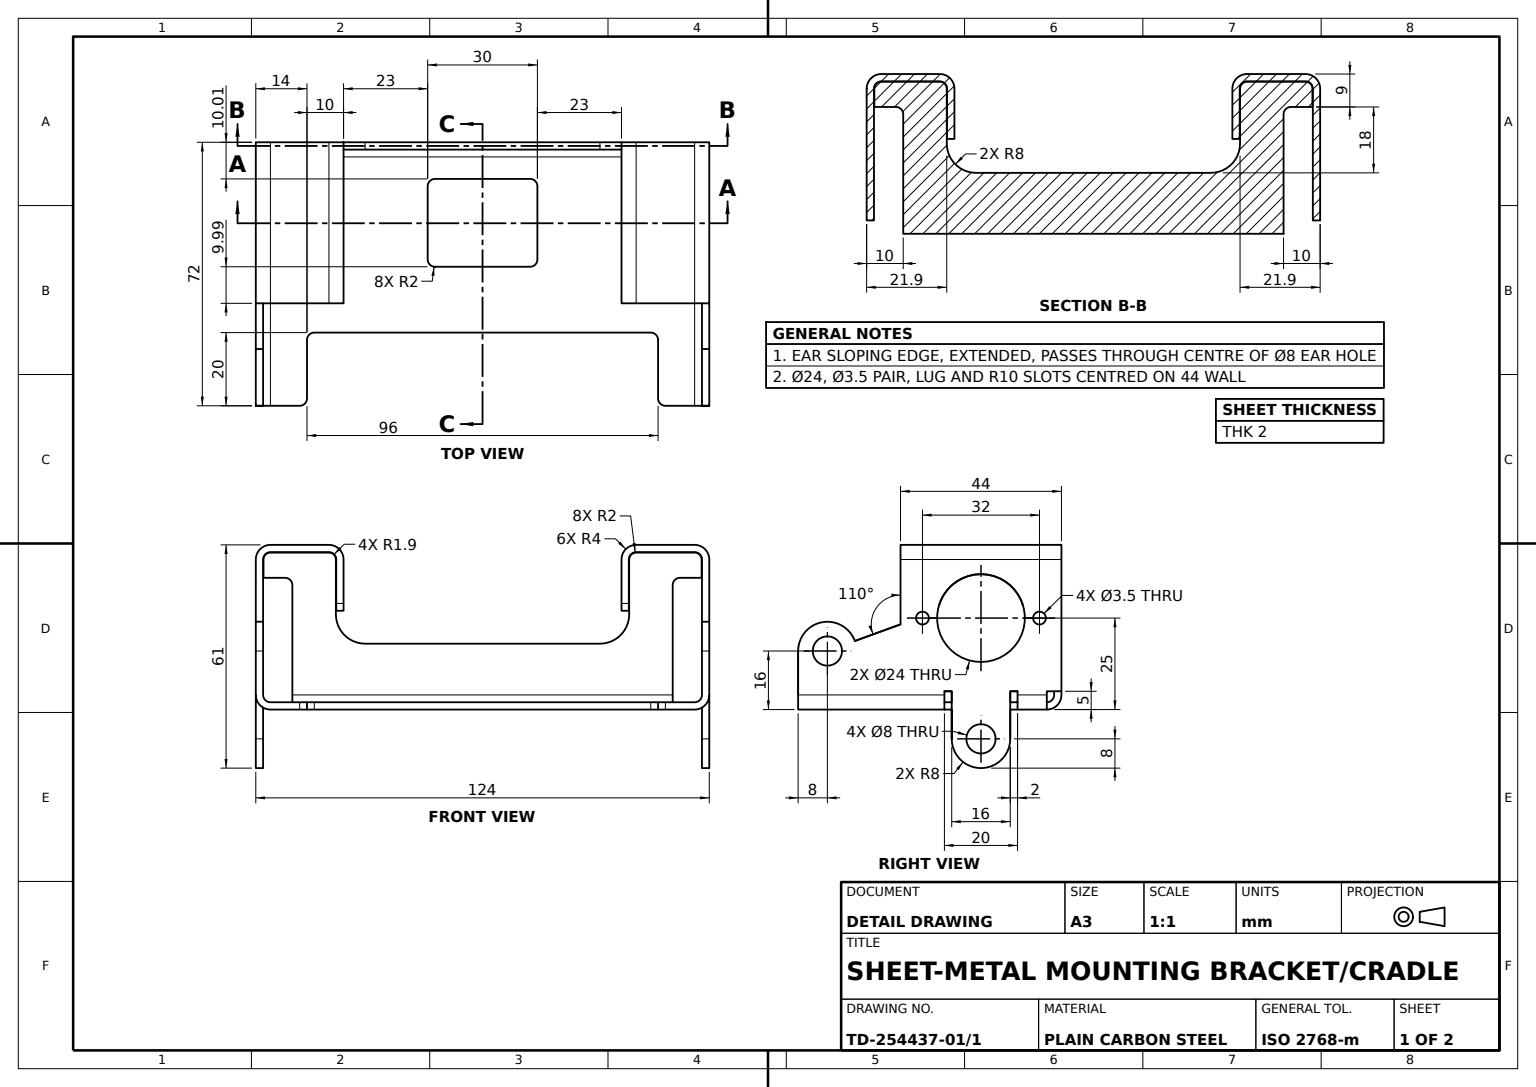
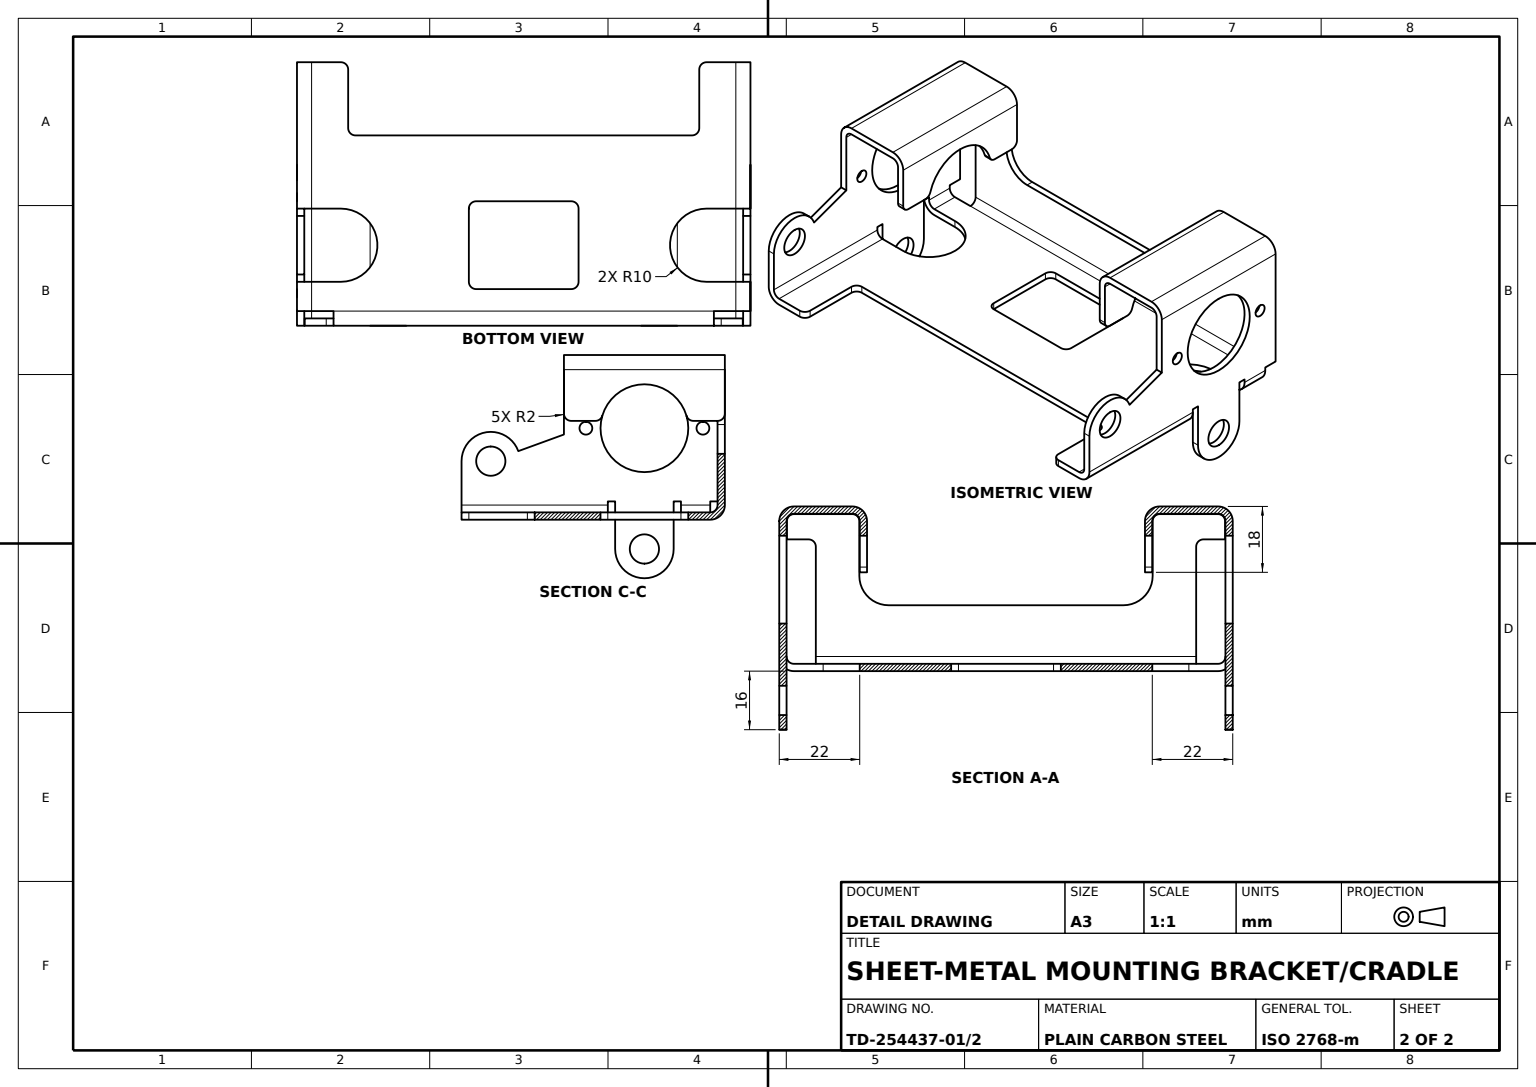
solid
v1 (42,43,0)
v2 (58,43,0)
e1 v1 v2 LINE
v3 (58,41,0)
e2 v3 v2 LINE
v4 (42,41,0)
e3 v4 v3 LINE
e4 v4 v1 LINE
face PLANE(AX(P(60,43,0),D(0,0,-1),D(-1,0,0))) [e1 -e2 -e3 e4]
v5 (48,0,54)
v6 (48,0,70)
e5 v5 v6 LINE
v7 (50,0,72)
e6 v6 v7 CIRCLE(AX(P(50,0,70),D(0,1,0),D(0,0,-1)),2)
v8 (58,0,72)
e7 v7 v8 LINE
v9 (58,0,32)
e8 v9 v8 LINE
v10 (50,0,32)
e9 v10 v9 LINE
v11 (50,0,12)
e10 v11 v10 CIRCLE(AX(P(50,0,22),D(0,1,0),D(0,0,-1)),10)
v12 (58,0,12)
e11 v12 v11 LINE
v13 (58,0,4)
e12 v13 v12 LINE
v14 (52,0,4)
e13 v13 v14 LINE
v15 (-52,0,4)
e14 v15 v14 LINE
v16 (-58,0,4)
e15 v15 v16 LINE
v17 (-58,0,12)
e16 v17 v16 LINE
v18 (-50,0,12)
e17 v18 v17 LINE
v19 (-50,0,32)
e18 v19 v18 CIRCLE(AX(P(-50,0,22),D(0,1,0),D(0,0,-1)),10)
v20 (-58,0,32)
e19 v20 v19 LINE
v21 (-58,0,72)
e20 v21 v20 LINE
v22 (-50,0,72)
e21 v21 v22 LINE
v23 (-48,0,70)
e22 v22 v23 CIRCLE(AX(P(-50,0,70),D(0,1,0),D(0,0,-1)),2)
v24 (-48,0,54)
e23 v23 v24 LINE
v25 (-46,0,52)
e24 v24 v25 CIRCLE(AX(P(-46,0,54),D(0,-1,0),D(0,0,1)),2)
v26 (46,0,52)
e25 v25 v26 LINE
e26 v26 v5 CIRCLE(AX(P(46,0,54),D(0,-1,0),D(0,0,1)),2)
v27 (15,0,32.008422)
v28 (15,0,12.008422)
e27 v27 v28 LINE
v29 (13,0,34.008422)
e28 v29 v27 CIRCLE(AX(P(13,0,32.008422),D(0,1,0),D(0,0,1)),2)
v30 (-13,0,34.008422)
e29 v30 v29 LINE
v31 (-15,0,32.008422)
e30 v31 v30 CIRCLE(AX(P(-13,0,32.008422),D(0,1,0),D(0,0,-1)),2)
v32 (-15,0,12.008422)
e31 v32 v31 LINE
v33 (-13,0,10.008422)
e32 v33 v32 CIRCLE(AX(P(-13,0,12.008422),D(0,1,0),D(0,0,1)),2)
v34 (13,0,10.008422)
e33 v34 v33 LINE
e34 v28 v34 CIRCLE(AX(P(13,0,12.008422),D(0,1,0),D(0,0,-1)),2)
face PLANE(AX(P(50,0,70),D(0,-1,0),D(0,0,-1))) rev [e5 e6 e7 -e8 -e9 -e10 -e11 -e12 e13 -e14 e15 -e16 -e17 -e18 -e19 -e20 e21 e22 e23 e24 e25 e26] [-e27 -e28 -e29 -e30 -e31 -e32 -e33 -e34]
v35 (62,24.75,6)
v36 (60,24.75,6)
e35 v35 v36 LINE
v37 (60,21.25,6)
e36 v36 v37 CIRCLE(AX(P(60,23,6),D(-1,0,0),D(0,-1,0)),1.75)
v38 (62,21.25,6)
e37 v38 v37 LINE
e38 v35 v38 CIRCLE(AX(P(62,23,6),D(-1,0,0),D(0,-1,0)),1.75)
face CYL(AX(P(62,23,6),D(-1,0,0),D(0,-1,0)),1.75) rev [e35 e36 -e37 -e38]
v39 (-38,27,44)
v40 (-38,39,44)
e39 v39 v40 LINE
v41 (-40,39,44)
e40 v41 v40 LINE
v42 (-40,27,44)
e41 v42 v41 LINE
e42 v39 v42 LINE
face PLANE(AX(P(-38,41,44),D(0,0,1),D(1,0,0))) [e39 -e40 -e41 -e42]
v43 (38,26.428571,33.499778)
v44 (38,25,35.416408)
e43 v43 v44 CIRCLE(AX(P(38,27,35.416408),D(-1,0,0),D(0,1,0)),2)
v45 (40,26.428571,33.499778)
e44 v43 v45 LINE
v46 (40,25,35.416408)
e45 v45 v46 CIRCLE(AX(P(40,27,35.416408),D(-1,0,0),D(0,1,0)),2)
e46 v44 v46 LINE
face CYL(AX(P(38,27,35.416408),D(1,0,0),D(0,1,0)),2) [-e43 e44 e45 -e46]
v47 (60,21.25,38)
v48 (60,24.75,38)
e47 v47 v48 CIRCLE(AX(P(60,23,38),D(-1,0,0),D(0,-1,0)),1.75)
v49 (62,24.75,38)
e48 v49 v48 LINE
v50 (62,21.25,38)
e49 v50 v49 CIRCLE(AX(P(62,23,38),D(-1,0,0),D(0,-1,0)),1.75)
e50 v50 v47 LINE
face CYL(AX(P(62,23,38),D(-1,0,0),D(0,-1,0)),1.75) rev [e47 -e48 -e49 e50]
v51 (-60,22,64)
v52 (-60,16.736161,56.482459)
e51 v51 v52 CIRCLE(AX(P(-60,14,64),D(-1,0,0),D(0,1,0)),8)
v53 (-62,16.736161,56.482459)
e52 v53 v52 LINE
v54 (-62,22,64)
e53 v54 v53 CIRCLE(AX(P(-62,14,64),D(-1,0,0),D(0,1,0)),8)
e54 v54 v51 LINE
face CYL(AX(P(-62,14,64),D(1,0,0),D(0,1,0)),8) [e51 -e52 -e53 e54]
v55 (-58,41,0)
v56 (-58,41,44)
e55 v55 v56 LINE
v57 (-42,41,0)
e56 v57 v55 LINE
v58 (-42,41,44)
e57 v58 v57 LINE
e58 v56 v58 LINE
face PLANE(AX(P(0,41,0),D(0,-1,0),D(1,0,0))) [-e55 -e56 -e57 -e58]
v59 (-58,43,44)
v60 (-58,43,0)
e59 v59 v60 LINE
v61 (-62,39,0)
e60 v60 v61 CIRCLE(AX(P(-58,39,0),D(0,0,1),D(0,-1,0)),4)
v62 (-62,39,44)
e61 v62 v61 LINE
e62 v62 v59 CIRCLE(AX(P(-58,39,44),D(0,0,-1),D(0,1,0)),4)
face CYL(AX(P(-58,39,66.296801),D(0,0,-1),D(0,1,0)),4) [e59 e60 -e61 e62]
v63 (52,2,2)
e63 v14 v63 CIRCLE(AX(P(52,2,4),D(1,0,0),D(0,0,1)),2)
v64 (52,-2,4)
e64 v14 v64 LINE
v65 (52,2,0)
e65 v64 v65 CIRCLE(AX(P(52,2,4),D(1,0,0),D(0,0,1)),4)
e66 v63 v65 LINE
face PLANE(AX(P(52,2,4),D(1,0,0),D(0,0,-1))) [-e63 e64 e65 -e66]
v66 (-40.1,39,0)
v67 (-40.1,39,2)
e67 v66 v67 LINE
v68 (-40.1,24,2)
e68 v67 v68 LINE
v69 (-40.1,24,0)
e69 v69 v68 LINE
e70 v66 v69 LINE
face PLANE(AX(P(-40.1,24,0),D(-1,0,0),D(0,-1,0))) rev [e67 e68 -e69 -e70]
v70 (62,35,22)
v71 (60,35,22)
e71 v70 v71 LINE
v72 (60,11,22)
e72 v71 v72 CIRCLE(AX(P(60,23,22),D(-1,0,0),D(0,-1,0)),12)
v73 (62,11,22)
e73 v73 v72 LINE
e74 v70 v73 CIRCLE(AX(P(62,23,22),D(-1,0,0),D(0,-1,0)),12)
face CYL(AX(P(62,23,22),D(-1,0,0),D(0,-1,0)),12) rev [e71 e72 -e73 -e74]
v74 (42,43,44)
e75 v1 v74 LINE
v75 (38,39,0)
e76 v1 v75 CIRCLE(AX(P(42,39,0),D(0,0,1),D(-1,0,0)),4)
v76 (38,39,44)
e77 v75 v76 LINE
e78 v76 v74 CIRCLE(AX(P(42,39,44),D(0,0,-1),D(1,0,0)),4)
face CYL(AX(P(42,39,-22.296801),D(0,0,1),D(-1,0,0)),4) [-e75 e76 e77 e78]
v77 (-38,25,2)
v78 (-40,25,2)
e79 v77 v78 LINE
v79 (-38,25,8.583592)
e80 v77 v79 LINE
v80 (-40,25,8.583592)
e81 v79 v80 LINE
e82 v78 v80 LINE
face PLANE(AX(P(-38,25,8.583592),D(0,-1,0),D(1,0,0))) [-e79 e80 e81 -e82]
v81 (40,39,0)
e83 v4 v81 CIRCLE(AX(P(42,39,0),D(0,0,1),D(-1,0,0)),2)
e84 v81 v75 LINE
face PLANE(AX(P(42,39,0),D(0,0,-1),D(1,0,0))) [-e4 e83 e84 -e76]
v82 (59.9,34,0)
v83 (59.9,34,2)
e85 v82 v83 LINE
v84 (54,34,2)
e86 v83 v84 LINE
v85 (54,34,0)
e87 v85 v84 LINE
e88 v82 v85 LINE
face PLANE(AX(P(59.9,34,0),D(0,1,0),D(0,0,1))) rev [e85 e86 -e87 -e88]
v86 (62,2,12)
v87 (60,2,12)
e89 v86 v87 LINE
v88 (62,3,12)
e90 v88 v86 LINE
v89 (60,3,12)
e91 v88 v89 LINE
e92 v89 v87 LINE
face PLANE(AX(P(62,3,12),D(0,0,-1),D(0,-1,0))) rev [-e89 -e90 e91 e92]
v90 (40,27,0)
v91 (40,25,2)
e93 v90 v91 CIRCLE(AX(P(40,27,2),D(-1,0,0),D(0,1,0)),2)
v92 (38,25,2)
e94 v92 v91 LINE
v93 (38,27,0)
e95 v93 v92 CIRCLE(AX(P(38,27,2),D(-1,0,0),D(0,1,0)),2)
e96 v93 v90 LINE
face CYL(AX(P(38,27,2),D(1,0,0),D(0,1,0)),2) [e93 -e94 -e95 e96]
v94 (-62,3,4)
v95 (-60,3,4)
e97 v94 v95 LINE
v96 (-60,2,4)
e98 v95 v96 LINE
v97 (-62,2,4)
e99 v96 v97 LINE
e100 v94 v97 LINE
face PLANE(AX(P(-62,0,4),D(0,0,1),D(1,0,0))) rev [e97 e98 e99 -e100]
v98 (-62,11,22)
v99 (-60,11,22)
e101 v98 v99 LINE
v100 (-60,35,22)
e102 v100 v99 CIRCLE(AX(P(-60,23,22),D(-1,0,0),D(0,1,0)),12)
v101 (-62,35,22)
e103 v101 v100 LINE
e104 v101 v98 CIRCLE(AX(P(-62,23,22),D(-1,0,0),D(0,1,0)),12)
face CYL(AX(P(-62,23,22),D(1,0,0),D(0,1,0)),12) rev [e101 -e102 -e103 e104]
v102 (-42,43,44)
v103 (-42,43,0)
e105 v102 v103 LINE
e106 v103 v60 LINE
e107 v59 v102 LINE
face PLANE(AX(P(0,43,0),D(0,-1,0),D(1,0,0))) rev [e105 e106 -e59 e107]
v104 (38,25,42)
e108 v44 v104 LINE
v105 (40,25,42)
e109 v46 v105 LINE
e110 v104 v105 LINE
face PLANE(AX(P(38,25,42),D(0,1,0),D(-1,0,0))) rev [-e108 e46 e109 -e110]
v106 (40,39,44)
e111 v106 v76 LINE
v107 (42,41,44)
e112 v106 v107 CIRCLE(AX(P(42,39,44),D(0,0,-1),D(-1,0,0)),2)
e113 v107 v74 LINE
face PLANE(AX(P(42,39,44),D(0,0,1),D(-1,0,0))) [-e111 e112 e113 -e78]
v108 (62,-10,14)
v109 (62,3,14)
e114 v108 v109 LINE
v110 (60,-10,14)
e115 v110 v108 LINE
v111 (60,3,14)
e116 v110 v111 LINE
e117 v111 v109 LINE
face PLANE(AX(P(60,-10,14),D(0,0,-1),D(0,1,0))) [-e114 -e115 e116 e117]
v112 (-62,14,72)
v113 (-60,14,72)
e118 v112 v113 LINE
e119 v113 v51 CIRCLE(AX(P(-60,14,64),D(-1,0,0),D(0,1,0)),8)
e120 v112 v54 CIRCLE(AX(P(-62,14,64),D(-1,0,0),D(0,1,0)),8)
face CYL(AX(P(-62,14,64),D(1,0,0),D(0,1,0)),8) [e118 e119 -e54 -e120]
e121 v106 v81 LINE
e122 v4 v107 LINE
face CYL(AX(P(42,39,-22.296801),D(0,0,1),D(-1,0,0)),2) rev [e121 -e83 e122 -e112]
v114 (-60,3,14)
v115 (-60,-10,14)
e123 v114 v115 LINE
v116 (-62,-10,14)
e124 v115 v116 LINE
v117 (-62,3,14)
e125 v117 v116 LINE
e126 v114 v117 LINE
face PLANE(AX(P(-60,3,14),D(0,0,-1),D(0,1,0))) [e123 e124 -e125 -e126]
v118 (40,35,22)
e127 v118 v45 CIRCLE(AX(P(40,23,22),D(1,0,0),D(0,1,0)),12)
v119 (38,35,22)
e128 v119 v43 CIRCLE(AX(P(38,23,22),D(1,0,0),D(0,1,0)),12)
e129 v119 v118 LINE
face CYL(AX(P(38,23,22),D(1,0,0),D(0,1,0)),12) rev [e127 -e44 -e128 e129]
v120 (50,-2,32)
e130 v120 v10 LINE
v121 (58,-2,32)
e131 v121 v9 LINE
e132 v120 v121 LINE
face PLANE(AX(P(63.712389,-2,32),D(0,0,1),D(1,0,0))) rev [e130 e9 -e131 -e132]
v122 (-52,2,2)
e133 v122 v15 CIRCLE(AX(P(-52,2,4),D(-1,0,0),D(0,0,1)),2)
v123 (-52,2,0)
e134 v122 v123 LINE
v124 (-52,-2,4)
e135 v123 v124 CIRCLE(AX(P(-52,2,4),D(-1,0,0),D(0,0,1)),4)
e136 v15 v124 LINE
face PLANE(AX(P(-52,2,4),D(1,0,0),D(0,0,-1))) rev [-e133 e134 e135 -e136]
v125 (-60,3,30)
v126 (-60,3,32)
e137 v125 v126 LINE
v127 (-62,3,32)
e138 v127 v126 LINE
v128 (-62,3,30)
e139 v128 v127 LINE
e140 v125 v128 LINE
face PLANE(AX(P(-62,3,12),D(0,1,0),D(0,0,1))) rev [e137 -e138 -e139 -e140]
v129 (-62,2,32)
e141 v127 v129 LINE
v130 (-62,2,72)
e142 v130 v129 LINE
e143 v130 v112 LINE
v131 (-62,21.279405,44)
e144 v53 v131 LINE
e145 v131 v62 LINE
v132 (-62,3,0)
e146 v61 v132 LINE
e147 v132 v94 LINE
v133 (-62,2,12)
e148 v133 v97 LINE
v134 (-62,3,12)
e149 v133 v134 LINE
e150 v134 v117 LINE
v135 (-62,-18,22)
e151 v116 v135 CIRCLE(AX(P(-62,-10,22),D(-1,0,0),D(0,-1,0)),8)
v136 (-62,-10,30)
e152 v135 v136 CIRCLE(AX(P(-62,-10,22),D(-1,0,0),D(0,-1,0)),8)
e153 v136 v128 LINE
v137 (-62,21.25,38)
v138 (-62,24.75,38)
e154 v137 v138 CIRCLE(AX(P(-62,23,38),D(-1,0,0),D(0,1,0)),1.75)
e155 v138 v137 CIRCLE(AX(P(-62,23,38),D(-1,0,0),D(0,1,0)),1.75)
v139 (-62,10,64)
v140 (-62,18,64)
e156 v139 v140 CIRCLE(AX(P(-62,14,64),D(-1,0,0),D(0,1,0)),4)
e157 v140 v139 CIRCLE(AX(P(-62,14,64),D(-1,0,0),D(0,1,0)),4)
v141 (-62,21.25,6)
v142 (-62,24.75,6)
e158 v141 v142 CIRCLE(AX(P(-62,23,6),D(-1,0,0),D(0,1,0)),1.75)
e159 v142 v141 CIRCLE(AX(P(-62,23,6),D(-1,0,0),D(0,1,0)),1.75)
e160 v98 v101 CIRCLE(AX(P(-62,23,22),D(-1,0,0),D(0,1,0)),12)
v143 (-62,-14,22)
v144 (-62,-6,22)
e161 v143 v144 CIRCLE(AX(P(-62,-10,22),D(-1,0,0),D(0,-1,0)),4)
e162 v144 v143 CIRCLE(AX(P(-62,-10,22),D(-1,0,0),D(0,-1,0)),4)
face PLANE(AX(P(-62,14,64),D(1,0,0),D(0,1,0))) rev [e139 e141 -e142 e143 e120 e53 e144 e145 e61 e146 e147 e100 -e148 e149 e150 e125 e151 e152 e153] [-e154 -e155] [-e156 -e157] [-e158 -e159] [-e160 -e104] [-e161 -e162]
v145 (38,25,8.583592)
e163 v92 v145 LINE
v146 (40,25,8.583592)
e164 v91 v146 LINE
e165 v145 v146 LINE
face PLANE(AX(P(38,25,8.583592),D(0,1,0),D(-1,0,0))) rev [-e163 e94 e164 -e165]
v147 (-59.9,34,2)
v148 (-59.9,39,2)
e166 v147 v148 LINE
v149 (-59.9,39,0)
e167 v149 v148 LINE
v150 (-59.9,34,0)
e168 v150 v149 LINE
e169 v150 v147 LINE
face PLANE(AX(P(-59.9,39,0),D(1,0,0),D(0,0,-1))) rev [e166 -e167 -e168 e169]
v151 (-50,-2,32)
v152 (-50,-2,12)
e170 v151 v152 CIRCLE(AX(P(-50,-2,22),D(0,1,0),D(0,0,-1)),10)
e171 v151 v19 LINE
e172 v152 v18 LINE
face CYL(AX(P(-50,-2,22),D(0,1,0),D(0,0,1)),10) rev [-e170 e171 e18 -e172]
e173 v81 v90 LINE
e174 v75 v93 LINE
face PLANE(AX(P(38,27,0),D(0,0,1),D(0,-1,0))) rev [-e84 e173 -e96 -e174]
v153 (-60,-6,22)
v154 (-60,-14,22)
e175 v153 v154 CIRCLE(AX(P(-60,-10,22),D(-1,0,0),D(0,-1,0)),4)
e176 v153 v144 LINE
e177 v154 v143 LINE
face CYL(AX(P(-60,-10,22),D(-1,0,0),D(0,-1,0)),4) rev [-e175 e176 e162 -e177]
v155 (-60,39,44)
e178 v155 v62 LINE
e179 v155 v56 CIRCLE(AX(P(-58,39,44),D(0,0,-1),D(0,1,0)),2)
e180 v56 v59 LINE
face PLANE(AX(P(-58,39,44),D(0,0,1),D(0,-1,0))) [-e62 -e178 e179 e180]
v156 (59.9,39,0)
e181 v156 v82 LINE
v157 (59.9,39,2)
e182 v156 v157 LINE
e183 v157 v83 LINE
face PLANE(AX(P(59.9,39,0),D(-1,0,0),D(0,-1,0))) rev [-e85 -e181 e182 e183]
e184 v109 v88 LINE
e185 v111 v89 LINE
face PLANE(AX(P(62,3,12),D(0,1,0),D(0,0,-1))) rev [-e184 -e117 e185 -e91]
v158 (-60,21.279405,44)
e186 v52 v158 LINE
e187 v131 v158 LINE
face PLANE(AX(P(-62,21.279405,44),D(0,-0.939692621,-0.342020143),D(0,0.342020143,-0.939692621))) rev [e186 -e187 -e144 e52]
e188 v154 v153 CIRCLE(AX(P(-60,-10,22),D(-1,0,0),D(0,-1,0)),4)
face CYL(AX(P(-60,-10,22),D(-1,0,0),D(0,-1,0)),4) rev [-e176 -e188 e177 e161]
v159 (60,39,0)
e189 v159 v3 CIRCLE(AX(P(58,39,0),D(0,0,1),D(0,1,0)),2)
v160 (60,39,44)
e190 v159 v160 LINE
v161 (58,41,44)
e191 v161 v160 CIRCLE(AX(P(58,39,44),D(0,0,-1),D(0,1,0)),2)
e192 v161 v3 LINE
face CYL(AX(P(58,39,-22.296801),D(0,0,1),D(0,1,0)),2) rev [-e189 e190 -e191 e192]
e193 v73 v70 CIRCLE(AX(P(62,23,22),D(-1,0,0),D(0,-1,0)),12)
e194 v72 v71 CIRCLE(AX(P(60,23,22),D(-1,0,0),D(0,-1,0)),12)
face CYL(AX(P(62,23,22),D(-1,0,0),D(0,-1,0)),12) rev [-e71 -e193 e73 e194]
v162 (62,-14,22)
v163 (62,-6,22)
e195 v162 v163 CIRCLE(AX(P(62,-10,22),D(1,0,0),D(0,1,0)),4)
v164 (60,-6,22)
e196 v164 v163 LINE
v165 (60,-14,22)
e197 v165 v164 CIRCLE(AX(P(60,-10,22),D(1,0,0),D(0,1,0)),4)
e198 v165 v162 LINE
face CYL(AX(P(60,-10,22),D(1,0,0),D(0,1,0)),4) rev [e195 -e196 -e197 e198]
v166 (-40,26.428571,10.500222)
e199 v80 v166 CIRCLE(AX(P(-40,27,8.583592),D(-1,0,0),D(0,-1,0)),2)
v167 (-40,26.428571,33.499778)
e200 v166 v167 CIRCLE(AX(P(-40,23,22),D(1,0,0),D(0,-1,0)),12)
v168 (-40,25,35.416408)
e201 v167 v168 CIRCLE(AX(P(-40,27,35.416408),D(-1,0,0),D(0,-1,0)),2)
v169 (-40,25,42)
e202 v168 v169 LINE
e203 v169 v42 CIRCLE(AX(P(-40,27,42),D(-1,0,0),D(0,-1,0)),2)
v170 (-40,39,0)
e204 v170 v41 LINE
v171 (-40,27,0)
e205 v170 v171 LINE
e206 v171 v78 CIRCLE(AX(P(-40,27,2),D(-1,0,0),D(0,-1,0)),2)
face PLANE(AX(P(-40,27,42),D(-1,0,0),D(0,-1,0))) [e199 e200 e201 e202 e203 e41 -e204 e205 e206 e82]
v172 (58,-2,4)
e207 v13 v172 LINE
e208 v172 v64 LINE
face PLANE(AX(P(-62,-2,4),D(0,0,-1),D(-1,0,0))) [e207 e208 -e64 -e13]
v173 (-60,24.75,38)
e209 v138 v173 LINE
v174 (-60,21.25,38)
e210 v174 v173 CIRCLE(AX(P(-60,23,38),D(-1,0,0),D(0,1,0)),1.75)
e211 v137 v174 LINE
face CYL(AX(P(-62,23,38),D(1,0,0),D(0,1,0)),1.75) rev [e154 e209 -e210 -e211]
v175 (60,2,72)
v176 (62,2,72)
e212 v175 v176 LINE
e213 v175 v8 CIRCLE(AX(P(58,2,72),D(0,0,-1),D(1,0,0)),2)
v177 (58,-2,72)
e214 v8 v177 LINE
e215 v176 v177 CIRCLE(AX(P(58,2,72),D(0,0,-1),D(-1,0,0)),4)
face PLANE(AX(P(58,2,72),D(0,0,1),D(1,0,0))) [-e212 e213 e214 -e215]
v178 (-32.1,16,0)
v179 (-32.1,16,2)
e216 v178 v179 LINE
e217 v69 v178 CIRCLE(AX(P(-32.1,24,0),D(0,0,1),D(0,1,0)),8)
e218 v68 v179 CIRCLE(AX(P(-32.1,24,2),D(0,0,1),D(0,1,0)),8)
face CYL(AX(P(-32.1,24,0),D(0,0,1),D(0,-1,0)),8) rev [-e216 -e217 e69 e218]
v180 (32.1,16,0)
v181 (40.1,24,0)
e219 v180 v181 CIRCLE(AX(P(32.1,24,0),D(0,0,1),D(0,1,0)),8)
v182 (32.1,16,2)
e220 v180 v182 LINE
v183 (40.1,24,2)
e221 v182 v183 CIRCLE(AX(P(32.1,24,2),D(0,0,1),D(0,1,0)),8)
e222 v181 v183 LINE
face CYL(AX(P(32.1,24,0),D(0,0,1),D(0,-1,0)),8) rev [-e219 e220 e221 -e222]
v184 (58,40.9,0)
e223 v184 v156 CIRCLE(AX(P(58,39,0),D(0,0,-1),D(0,1,0)),1.9)
v185 (58,40.9,2)
e224 v184 v185 LINE
e225 v185 v157 CIRCLE(AX(P(58,39,2),D(0,0,-1),D(0,1,0)),1.9)
face CYL(AX(P(58,39,0),D(0,0,1),D(0,-1,0)),1.9) [-e182 -e223 e224 e225]
v186 (60,2,32)
v187 (62,2,32)
e226 v186 v187 LINE
e227 v121 v187 CIRCLE(AX(P(58,2,32),D(0,0,1),D(1,0,0)),4)
e228 v9 v186 CIRCLE(AX(P(58,2,32),D(0,0,1),D(1,0,0)),2)
face PLANE(AX(P(58,2,32),D(0,0,-1),D(-1,0,0))) [e226 -e227 e131 e228]
v188 (-42,40.9,0)
v189 (-42,40.9,2)
e229 v188 v189 LINE
v190 (-58,40.9,0)
e230 v190 v188 LINE
v191 (-58,40.9,2)
e231 v190 v191 LINE
e232 v191 v189 LINE
face PLANE(AX(P(-42,40.9,0),D(0,-1,0),D(1,0,0))) rev [-e229 -e230 e231 e232]
v192 (48,-2,70)
e233 v192 v6 LINE
v193 (50,-2,72)
e234 v192 v193 CIRCLE(AX(P(50,-2,70),D(0,1,0),D(0,0,-1)),2)
e235 v193 v7 LINE
face CYL(AX(P(50,-2,70),D(0,1,0),D(0,0,1)),2) [-e6 -e233 e234 e235]
v194 (62,14,72)
e236 v176 v194 LINE
v195 (60,14,72)
e237 v194 v195 LINE
e238 v175 v195 LINE
face PLANE(AX(P(62,14,72),D(0,0,1),D(1,0,0))) [e212 e236 e237 -e238]
v196 (-60,3,0)
e239 v196 v95 LINE
e240 v132 v196 LINE
face PLANE(AX(P(-62,3,4),D(0,1,0),D(-1,0,0))) rev [e239 -e97 -e147 e240]
v197 (-60,2,12)
e241 v17 v197 CIRCLE(AX(P(-58,2,12),D(0,0,-1),D(-1,0,0)),2)
e242 v96 v16 CIRCLE(AX(P(-58,2,4),D(0,0,1),D(-1,0,0)),2)
e243 v96 v197 LINE
face CYL(AX(P(-58,2,17.497716),D(0,0,-1),D(-1,0,0)),2) rev [-e241 e16 -e242 e243]
e244 v163 v162 CIRCLE(AX(P(62,-10,22),D(1,0,0),D(0,1,0)),4)
e245 v164 v165 CIRCLE(AX(P(60,-10,22),D(1,0,0),D(0,1,0)),4)
face CYL(AX(P(60,-10,22),D(1,0,0),D(0,1,0)),4) rev [e196 e244 -e198 -e245]
v198 (-54,34,2)
e246 v198 v147 LINE
v199 (-54,34,0)
e247 v199 v150 LINE
e248 v199 v198 LINE
face PLANE(AX(P(-59.9,34,0),D(0,1,0),D(0,0,1))) rev [e246 -e169 -e247 e248]
v200 (-52,32,2)
e249 v200 v198 CIRCLE(AX(P(-54,32,2),D(0,0,1),D(0,1,0)),2)
v201 (-52,32,0)
e250 v201 v199 CIRCLE(AX(P(-54,32,0),D(0,0,1),D(0,1,0)),2)
e251 v201 v200 LINE
face CYL(AX(P(-54,32,0),D(0,0,1),D(0,-1,0)),2) rev [e249 -e248 -e250 e251]
v202 (-58,-2,32)
e252 v129 v202 CIRCLE(AX(P(-58,2,32),D(0,0,1),D(1,0,0)),4)
v203 (-58,-2,72)
e253 v203 v202 LINE
e254 v203 v130 CIRCLE(AX(P(-58,2,72),D(0,0,-1),D(-1,0,0)),4)
face CYL(AX(P(-58,2,92.326252),D(0,0,-1),D(-1,0,0)),4) [e142 e252 -e253 e254]
v204 (-60,21.25,6)
e255 v141 v204 LINE
v205 (-60,24.75,6)
e256 v142 v205 LINE
e257 v204 v205 CIRCLE(AX(P(-60,23,6),D(-1,0,0),D(0,1,0)),1.75)
face CYL(AX(P(-62,23,6),D(1,0,0),D(0,1,0)),1.75) rev [-e255 e158 e256 -e257]
v206 (-58,-2,4)
e258 v16 v206 LINE
e259 v97 v206 CIRCLE(AX(P(-58,2,4),D(0,0,1),D(0,-1,0)),4)
face PLANE(AX(P(-58,2,4),D(0,0,-1),D(0,1,0))) [e242 e258 -e259 -e99]
v207 (-60,39,0)
e260 v207 v61 LINE
e261 v207 v196 LINE
face PLANE(AX(P(-62,3,0),D(0,0,1),D(1,0,0))) rev [-e146 -e260 e261 -e240]
e262 v179 v182 LINE
e263 v178 v180 LINE
face PLANE(AX(P(32.1,16,0),D(0,-1,0),D(0,0,-1))) rev [e216 e262 -e220 -e263]
e264 v38 v35 CIRCLE(AX(P(62,23,6),D(-1,0,0),D(0,-1,0)),1.75)
e265 v37 v36 CIRCLE(AX(P(60,23,6),D(-1,0,0),D(0,-1,0)),1.75)
face CYL(AX(P(62,23,6),D(-1,0,0),D(0,-1,0)),1.75) rev [-e264 e37 e265 -e35]
v208 (62,16.736161,56.482459)
v209 (60,16.736161,56.482459)
e266 v208 v209 LINE
v210 (62,21.279405,44)
e267 v208 v210 LINE
v211 (60,21.279405,44)
e268 v210 v211 LINE
e269 v209 v211 LINE
face PLANE(AX(P(62,21.279405,44),D(0,0.939692621,0.342020143),D(0,-0.342020143,0.939692621))) [-e266 e267 e268 -e269]
v212 (13,-2,34.008422)
e270 v212 v29 LINE
v213 (-13,-2,34.008422)
e271 v213 v212 LINE
e272 v213 v30 LINE
face PLANE(AX(P(-13,-2,34.008422),D(0,0,1),D(1,0,0))) rev [e29 -e270 -e271 e272]
e273 v124 v206 LINE
face PLANE(AX(P(-62,-2,4),D(0,0,-1),D(-1,0,0))) [e136 e273 -e258 -e15]
v214 (60,-10,30)
e274 v214 v110 CIRCLE(AX(P(60,-10,22),D(1,0,0),D(0,1,0)),8)
v215 (62,-10,30)
e275 v215 v108 CIRCLE(AX(P(62,-10,22),D(1,0,0),D(0,1,0)),8)
e276 v214 v215 LINE
face CYL(AX(P(60,-10,22),D(1,0,0),D(0,1,0)),8) [e274 e115 -e275 -e276]
v216 (-38,26.428571,33.499778)
e277 v216 v167 LINE
v217 (-38,25,35.416408)
e278 v216 v217 CIRCLE(AX(P(-38,27,35.416408),D(-1,0,0),D(0,-1,0)),2)
e279 v217 v168 LINE
face CYL(AX(P(-38,27,35.416408),D(-1,0,0),D(0,-1,0)),2) [-e201 -e277 e278 e279]
v218 (-38,25,42)
e280 v218 v169 LINE
e281 v217 v218 LINE
face PLANE(AX(P(-38,25,42),D(0,-1,0),D(1,0,0))) [e280 -e202 -e279 e281]
v219 (52,32,2)
e282 v84 v219 CIRCLE(AX(P(54,32,2),D(0,0,1),D(0,1,0)),2)
v220 (52,32,0)
e283 v220 v219 LINE
e284 v85 v220 CIRCLE(AX(P(54,32,0),D(0,0,1),D(0,1,0)),2)
face CYL(AX(P(54,32,0),D(0,0,1),D(0,-1,0)),2) rev [e87 e282 -e283 -e284]
v221 (60,3,30)
e285 v221 v214 LINE
v222 (62,3,30)
e286 v222 v215 LINE
e287 v221 v222 LINE
face PLANE(AX(P(60,3,30),D(0,0,1),D(1,0,0))) [e285 e276 -e286 -e287]
v223 (-60,2,32)
e288 v129 v223 LINE
e289 v126 v223 LINE
face PLANE(AX(P(-62,3,32),D(0,0,1),D(0,-1,0))) rev [-e288 -e141 e138 e289]
v224 (13,-2,10.008422)
e290 v224 v34 LINE
v225 (15,-2,12.008422)
e291 v225 v224 CIRCLE(AX(P(13,-2,12.008422),D(0,1,0),D(0,0,-1)),2)
e292 v225 v28 LINE
face CYL(AX(P(13,-2,12.008422),D(0,1,0),D(0,0,1)),2) rev [e34 -e290 -e291 e292]
v226 (62,39,0)
e293 v226 v2 CIRCLE(AX(P(58,39,0),D(0,0,1),D(0,1,0)),4)
e294 v159 v226 LINE
face PLANE(AX(P(58,39,0),D(0,0,-1),D(0,-1,0))) [e189 e2 -e293 -e294]
e295 v63 v122 LINE
face CYL(AX(P(-52,2,4),D(-1,0,0),D(0,0,-1)),2) rev [e133 e14 e63 e295]
v227 (-38,27,0)
e296 v227 v171 LINE
e297 v227 v77 CIRCLE(AX(P(-38,27,2),D(-1,0,0),D(0,-1,0)),2)
face CYL(AX(P(-38,27,2),D(-1,0,0),D(0,-1,0)),2) [-e206 -e296 e297 e79]
v228 (62,10,64)
v229 (62,18,64)
e298 v228 v229 CIRCLE(AX(P(62,14,64),D(-1,0,0),D(0,-1,0)),4)
v230 (60,10,64)
e299 v228 v230 LINE
v231 (60,18,64)
e300 v230 v231 CIRCLE(AX(P(60,14,64),D(-1,0,0),D(0,-1,0)),4)
e301 v229 v231 LINE
face CYL(AX(P(62,14,64),D(-1,0,0),D(0,-1,0)),4) rev [-e298 e299 e300 -e301]
e302 v49 v50 CIRCLE(AX(P(62,23,38),D(-1,0,0),D(0,-1,0)),1.75)
e303 v48 v47 CIRCLE(AX(P(60,23,38),D(-1,0,0),D(0,-1,0)),1.75)
face CYL(AX(P(62,23,38),D(-1,0,0),D(0,-1,0)),1.75) rev [-e302 e48 e303 -e50]
v232 (62,39,44)
e304 v210 v232 LINE
e305 v160 v232 LINE
e306 v211 v160 LINE
face PLANE(AX(P(62,43,44),D(0,0,1),D(1,0,0))) [-e268 e304 -e305 -e306]
e307 v58 v102 LINE
face PLANE(AX(P(-38,43,44),D(0,0,-1),D(-1,0,0))) rev [e58 e307 -e107 -e180]
e308 v21 v203 LINE
v233 (-60,2,72)
e309 v21 v233 CIRCLE(AX(P(-58,2,72),D(0,0,-1),D(-1,0,0)),2)
e310 v233 v130 LINE
face PLANE(AX(P(-58,2,72),D(0,0,1),D(1,0,0))) [-e308 e309 e310 -e254]
e311 v175 v186 LINE
face CYL(AX(P(58,2,11.673748),D(0,0,1),D(1,0,0)),2) rev [e311 -e228 e8 -e213]
v234 (46,-2,52)
e312 v234 v26 LINE
v235 (-46,-2,52)
e313 v235 v25 LINE
e314 v235 v234 LINE
face PLANE(AX(P(46,-2,52),D(0,0,1),D(1,0,0))) [e312 -e25 -e313 e314]
e315 v55 v207 CIRCLE(AX(P(-58,39,0),D(0,0,1),D(0,1,0)),2)
e316 v55 v60 LINE
face PLANE(AX(P(-58,39,0),D(0,0,-1),D(0,1,0))) [e315 e260 -e60 -e316]
e317 v233 v113 LINE
face PLANE(AX(P(-62,14,72),D(0,0,-1),D(-1,0,0))) rev [-e118 -e143 -e310 e317]
e318 v57 v103 LINE
face PLANE(AX(P(-60,43,0),D(0,0,1),D(1,0,0))) rev [-e318 e56 e316 -e106]
e319 v161 v107 LINE
v236 (58,43,44)
e320 v161 v236 LINE
e321 v236 v74 LINE
face PLANE(AX(P(38,43,44),D(0,0,1),D(1,0,0))) [-e113 -e319 e320 e321]
v237 (40,27,44)
e322 v237 v106 LINE
v238 (38,27,44)
e323 v238 v76 LINE
e324 v238 v237 LINE
face PLANE(AX(P(38,41,44),D(0,0,-1),D(-1,0,0))) rev [e322 e111 -e323 e324]
v239 (-38,39,0)
e325 v239 v227 LINE
e326 v40 v239 LINE
e327 v218 v39 CIRCLE(AX(P(-38,27,42),D(-1,0,0),D(0,-1,0)),2)
v240 (-38,26.428571,10.500222)
e328 v240 v216 CIRCLE(AX(P(-38,23,22),D(1,0,0),D(0,-1,0)),12)
e329 v79 v240 CIRCLE(AX(P(-38,27,8.583592),D(-1,0,0),D(0,-1,0)),2)
face PLANE(AX(P(-38,27,42),D(-1,0,0),D(0,-1,0))) rev [-e80 -e297 -e325 -e326 -e39 -e327 -e281 -e278 -e328 -e329]
v241 (60,2,4)
e330 v13 v241 CIRCLE(AX(P(58,2,4),D(0,0,1),D(1,0,0)),2)
e331 v87 v12 CIRCLE(AX(P(58,2,12),D(0,0,-1),D(1,0,0)),2)
e332 v87 v241 LINE
face CYL(AX(P(58,2,-1.497716),D(0,0,1),D(1,0,0)),2) rev [-e330 e12 -e331 e332]
v242 (-60,-10,30)
e333 v242 v125 LINE
e334 v242 v136 LINE
face PLANE(AX(P(-60,3,30),D(0,0,1),D(1,0,0))) [e333 e140 -e153 -e334]
face PLANE(AX(P(0,41,0),D(0,-1,0),D(-1,0,0))) [-e192 e319 -e122 e3]
e335 v223 v20 CIRCLE(AX(P(-58,2,32),D(0,0,1),D(-1,0,0)),2)
e336 v223 v233 LINE
face CYL(AX(P(-58,2,92.326252),D(0,0,-1),D(-1,0,0)),2) rev [e20 -e335 e336 -e309]
e337 v20 v202 LINE
face PLANE(AX(P(-58,2,32),D(0,0,-1),D(-1,0,0))) [e288 e335 e337 -e252]
e338 v229 v228 CIRCLE(AX(P(62,14,64),D(-1,0,0),D(0,-1,0)),4)
e339 v187 v176 LINE
v243 (62,3,32)
e340 v187 v243 LINE
e341 v243 v222 LINE
v244 (62,2,4)
e342 v244 v86 LINE
v245 (62,3,4)
e343 v245 v244 LINE
v246 (62,3,0)
e344 v246 v245 LINE
e345 v226 v246 LINE
e346 v226 v232 LINE
e347 v194 v208 CIRCLE(AX(P(62,14,64),D(-1,0,0),D(0,-1,0)),8)
face PLANE(AX(P(62,14,64),D(-1,0,0),D(0,1,0))) rev [e298 e338] [e74 e193] [e49 e302] [e38 e264] [-e244 -e195] [-e339 e340 e341 e286 e275 e114 e184 e90 -e342 -e343 -e344 -e345 e346 -e304 -e267 -e347 -e236]
v247 (-15,-2,12.008422)
v248 (-15,-2,32.008422)
e348 v247 v248 LINE
e349 v247 v32 LINE
e350 v248 v31 LINE
face PLANE(AX(P(-15,-2,32.008422),D(-1,0,0),D(0,0,1))) rev [-e348 e349 e31 -e350]
v249 (40,26.428571,10.500222)
e351 v249 v118 CIRCLE(AX(P(40,23,22),D(1,0,0),D(0,1,0)),12)
v250 (38,26.428571,10.500222)
e352 v250 v119 CIRCLE(AX(P(38,23,22),D(1,0,0),D(0,1,0)),12)
e353 v250 v249 LINE
face CYL(AX(P(38,23,22),D(1,0,0),D(0,1,0)),12) rev [e351 -e129 -e352 e353]
e354 v2 v236 LINE
face PLANE(AX(P(0,43,0),D(0,-1,0),D(-1,0,0))) rev [-e1 e75 -e321 -e354]
v251 (-60,10,64)
v252 (-60,18,64)
e355 v251 v252 CIRCLE(AX(P(-60,14,64),D(-1,0,0),D(0,1,0)),4)
e356 v139 v251 LINE
e357 v140 v252 LINE
face CYL(AX(P(-62,14,64),D(1,0,0),D(0,1,0)),4) rev [-e355 -e356 e156 e357]
e358 v205 v204 CIRCLE(AX(P(-60,23,6),D(-1,0,0),D(0,1,0)),1.75)
face CYL(AX(P(-62,23,6),D(1,0,0),D(0,1,0)),1.75) rev [e159 e255 -e358 -e256]
e359 v220 v65 LINE
e360 v219 v63 LINE
face PLANE(AX(P(52,0,0),D(-1,0,0),D(0,0,1))) rev [-e359 e283 e360 e66]
e361 v195 v209 CIRCLE(AX(P(60,14,64),D(-1,0,0),D(0,-1,0)),8)
face CYL(AX(P(62,14,64),D(-1,0,0),D(0,-1,0)),8) [e266 -e361 -e237 e347]
e362 v197 v133 LINE
v253 (-60,3,12)
e363 v197 v253 LINE
e364 v134 v253 LINE
face PLANE(AX(P(-62,3,12),D(0,0,-1),D(0,1,0))) rev [-e149 -e362 e363 -e364]
v254 (60,3,32)
e365 v186 v254 LINE
e366 v243 v254 LINE
face PLANE(AX(P(62,3,32),D(0,0,1),D(0,1,0))) rev [e365 -e366 -e340 -e226]
e367 v65 v123 LINE
e368 v124 v64 LINE
face CYL(AX(P(-52,2,4),D(-1,0,0),D(0,0,-1)),4) [-e135 -e367 -e65 -e368]
e369 v239 v103 CIRCLE(AX(P(-42,39,0),D(0,0,1),D(-1,0,0)),4)
e370 v102 v40 CIRCLE(AX(P(-42,39,44),D(0,0,-1),D(1,0,0)),4)
face CYL(AX(P(-42,39,66.296801),D(0,0,-1),D(1,0,0)),4) [e326 e369 -e105 e370]
e371 v248 v213 CIRCLE(AX(P(-13,-2,32.008422),D(0,1,0),D(0,0,-1)),2)
face CYL(AX(P(-13,-2,32.008422),D(0,1,0),D(0,0,1)),2) rev [e350 e30 -e272 -e371]
e372 v240 v166 LINE
face CYL(AX(P(-38,27,8.583592),D(-1,0,0),D(0,-1,0)),2) [-e199 -e81 e329 e372]
v255 (-48,-2,54)
e373 v255 v235 CIRCLE(AX(P(-46,-2,54),D(0,-1,0),D(0,0,1)),2)
v256 (-48,-2,70)
e374 v256 v255 LINE
v257 (-50,-2,72)
e375 v257 v256 CIRCLE(AX(P(-50,-2,70),D(0,1,0),D(0,0,-1)),2)
e376 v203 v257 LINE
e377 v202 v151 LINE
v258 (-58,-2,12)
e378 v152 v258 LINE
e379 v258 v206 LINE
v259 (58,-2,12)
e380 v172 v259 LINE
v260 (50,-2,12)
e381 v259 v260 LINE
e382 v260 v120 CIRCLE(AX(P(50,-2,22),D(0,1,0),D(0,0,-1)),10)
e383 v121 v177 LINE
e384 v193 v177 LINE
v261 (48,-2,54)
e385 v261 v192 LINE
e386 v234 v261 CIRCLE(AX(P(46,-2,54),D(0,-1,0),D(0,0,1)),2)
v262 (-13,-2,10.008422)
e387 v262 v247 CIRCLE(AX(P(-13,-2,12.008422),D(0,1,0),D(0,0,1)),2)
v263 (15,-2,32.008422)
e388 v212 v263 CIRCLE(AX(P(13,-2,32.008422),D(0,1,0),D(0,0,1)),2)
e389 v263 v225 LINE
e390 v224 v262 LINE
face PLANE(AX(P(50,-2,70),D(0,-1,0),D(0,0,-1))) [-e314 -e373 -e374 -e375 -e376 e253 e377 e170 e378 e379 -e273 e368 -e208 e380 e381 e382 e132 e383 -e384 -e234 -e385 -e386] [e387 e348 e371 e271 e388 e389 e291 e390]
face CYL(AX(P(-38,23,22),D(-1,0,0),D(0,-1,0)),12) rev [-e372 e328 e277 -e200]
e391 v236 v232 CIRCLE(AX(P(58,39,44),D(0,0,-1),D(0,-1,0)),4)
face PLANE(AX(P(58,39,44),D(0,0,1),D(0,1,0))) [-e391 -e320 e191 e305]
e392 v173 v174 CIRCLE(AX(P(-60,23,38),D(-1,0,0),D(0,1,0)),1.75)
face CYL(AX(P(-62,23,38),D(1,0,0),D(0,1,0)),1.75) rev [e211 -e392 -e209 e155]
e393 v155 v207 LINE
face CYL(AX(P(-58,39,66.296801),D(0,0,-1),D(0,1,0)),2) rev [e393 -e315 e55 -e179]
e394 v258 v133 CIRCLE(AX(P(-58,2,12),D(0,0,-1),D(-1,0,0)),4)
face CYL(AX(P(-58,2,17.497716),D(0,0,-1),D(-1,0,0)),4) [e148 e259 -e379 e394]
e395 v254 v221 LINE
face PLANE(AX(P(62,3,12),D(0,1,0),D(0,0,-1))) rev [e395 e287 -e341 e366]
face CYL(AX(P(-38,27,42),D(-1,0,0),D(0,-1,0)),2) [-e280 e327 e42 -e203]
e396 v149 v190 CIRCLE(AX(P(-58,39,0),D(0,0,-1),D(0,1,0)),1.9)
e397 v148 v191 CIRCLE(AX(P(-58,39,2),D(0,0,-1),D(0,1,0)),1.9)
face CYL(AX(P(-58,39,0),D(0,0,1),D(0,-1,0)),1.9) [-e396 e167 e397 -e231]
v264 (42,40.9,0)
v265 (42,40.9,2)
e398 v264 v265 LINE
v266 (40.1,39,0)
e399 v266 v264 CIRCLE(AX(P(42,39,0),D(0,0,-1),D(0,1,0)),1.9)
v267 (40.1,39,2)
e400 v266 v267 LINE
e401 v267 v265 CIRCLE(AX(P(42,39,2),D(0,0,-1),D(0,1,0)),1.9)
face CYL(AX(P(42,39,0),D(0,0,1),D(0,-1,0)),1.9) [-e398 -e399 e400 e401]
e402 v262 v33 LINE
face CYL(AX(P(-13,-2,12.008422),D(0,1,0),D(0,0,1)),2) rev [-e349 -e387 e402 e32]
e403 v264 v184 LINE
e404 v265 v185 LINE
face PLANE(AX(P(42,40.9,0),D(0,-1,0),D(1,0,0))) rev [-e224 -e403 e398 e404]
e405 v252 v251 CIRCLE(AX(P(-60,14,64),D(-1,0,0),D(0,1,0)),4)
e406 v99 v100 CIRCLE(AX(P(-60,23,22),D(-1,0,0),D(0,1,0)),12)
e407 v158 v155 LINE
v268 (-60,-18,22)
e408 v268 v242 CIRCLE(AX(P(-60,-10,22),D(-1,0,0),D(0,-1,0)),8)
e409 v115 v268 CIRCLE(AX(P(-60,-10,22),D(-1,0,0),D(0,-1,0)),8)
e410 v253 v114 LINE
face PLANE(AX(P(-60,14,64),D(1,0,0),D(0,1,0))) [e175 e188] [e355 e405] [e102 e406] [e358 e257] [-e363 -e243 -e98 -e239 -e261 -e393 -e407 -e186 -e51 -e119 -e317 -e336 -e289 -e137 -e333 -e408 -e409 -e123 -e410] [e210 e392]
e411 v257 v22 LINE
face PLANE(AX(P(-50,-2,72),D(0,0,1),D(1,0,0))) [e411 -e21 e308 e376]
e412 v145 v250 CIRCLE(AX(P(38,27,8.583592),D(-1,0,0),D(0,1,0)),2)
e413 v146 v249 CIRCLE(AX(P(40,27,8.583592),D(-1,0,0),D(0,1,0)),2)
face CYL(AX(P(38,27,8.583592),D(1,0,0),D(0,1,0)),2) [-e412 e165 e413 -e353]
e414 v170 v239 LINE
face PLANE(AX(P(-38,27,0),D(0,0,-1),D(0,1,0))) [e414 e325 e296 -e205]
e415 v172 v244 CIRCLE(AX(P(58,2,4),D(0,0,1),D(1,0,0)),4)
e416 v241 v244 LINE
face PLANE(AX(P(58,2,4),D(0,0,-1),D(-1,0,0))) [-e415 -e207 e330 e416]
e417 v170 v57 CIRCLE(AX(P(-42,39,0),D(0,0,1),D(1,0,0)),2)
face PLANE(AX(P(-42,39,0),D(0,0,-1),D(1,0,0))) [-e369 -e414 e417 e318]
e418 v260 v11 LINE
face CYL(AX(P(50,-2,22),D(0,1,0),D(0,0,1)),10) rev [e10 -e130 -e382 e418]
e419 v263 v27 LINE
face PLANE(AX(P(15,-2,32.008422),D(1,0,0),D(0,0,-1))) rev [-e389 e419 e27 -e292]
e420 v12 v259 LINE
e421 v86 v259 CIRCLE(AX(P(58,2,12),D(0,0,-1),D(-1,0,0)),4)
face PLANE(AX(P(58,2,12),D(0,0,1),D(1,0,0))) [e89 e331 e420 -e421]
e422 v58 v41 CIRCLE(AX(P(-42,39,44),D(0,0,-1),D(1,0,0)),2)
face PLANE(AX(P(-42,39,44),D(0,0,1),D(-1,0,0))) [-e370 -e307 e422 e40]
face PLANE(AX(P(-13,-2,10.008422),D(0,0,-1),D(-1,0,0))) rev [e290 e33 -e402 -e390]
e423 v255 v24 LINE
face CYL(AX(P(-46,-2,54),D(0,1,0),D(0,0,1)),2) rev [e373 e313 -e24 -e423]
e424 v122 v200 LINE
e425 v183 v267 LINE
e426 v189 v67 CIRCLE(AX(P(-42,39,2),D(0,0,-1),D(0,1,0)),1.9)
face PLANE(AX(P(54,32,2),D(0,0,-1),D(0,1,0))) rev [-e397 -e166 -e246 -e249 -e424 -e295 -e360 -e282 -e86 -e183 -e225 -e404 -e401 -e425 -e221 -e262 -e218 -e68 -e426 -e232]
e427 v268 v135 LINE
face CYL(AX(P(-60,-10,22),D(-1,0,0),D(0,-1,0)),8) [-e152 -e427 e408 e334]
v269 (60,3,0)
v270 (60,3,4)
e428 v269 v270 LINE
e429 v246 v269 LINE
e430 v245 v270 LINE
face PLANE(AX(P(62,3,4),D(0,-1,0),D(1,0,0))) [-e428 -e429 e344 e430]
face CYL(AX(P(58,2,11.673748),D(0,0,1),D(1,0,0)),4) [e227 e339 e215 -e383]
e431 v105 v237 CIRCLE(AX(P(40,27,42),D(-1,0,0),D(0,1,0)),2)
face PLANE(AX(P(40,27,42),D(1,0,0),D(0,-1,0))) [-e322 -e431 -e109 -e45 -e127 -e351 -e413 -e164 -e93 -e173 -e121]
e432 v188 v66 CIRCLE(AX(P(-42,39,0),D(0,0,-1),D(0,1,0)),1.9)
face CYL(AX(P(-42,39,0),D(0,0,1),D(0,-1,0)),1.9) [e229 e426 -e67 -e432]
e433 v104 v238 CIRCLE(AX(P(38,27,42),D(-1,0,0),D(0,1,0)),2)
face PLANE(AX(P(38,27,42),D(1,0,0),D(0,-1,0))) rev [-e77 e174 e95 e163 e412 e352 e128 e43 e108 e433 e323]
e434 v231 v230 CIRCLE(AX(P(60,14,64),D(-1,0,0),D(0,-1,0)),4)
face CYL(AX(P(62,14,64),D(-1,0,0),D(0,-1,0)),4) rev [-e338 e301 e434 -e299]
face PLANE(AX(P(-62,43,44),D(0,0,-1),D(-1,0,0))) rev [-e145 e187 e407 e178]
e435 v181 v266 LINE
face PLANE(AX(P(40.1,24,0),D(1,0,0),D(0,1,0))) rev [-e400 -e435 e222 e425]
e436 v159 v269 LINE
face PLANE(AX(P(62,3,0),D(0,0,-1),D(-1,0,0))) [e294 e345 e429 -e436]
e437 v123 v201 LINE
face PLANE(AX(P(-52,0,0),D(1,0,0),D(0,0,-1))) rev [-e134 e424 -e251 -e437]
face CYL(AX(P(-62,14,64),D(1,0,0),D(0,1,0)),4) rev [e356 -e405 -e357 e157]
face CYL(AX(P(-60,-10,22),D(-1,0,0),D(0,-1,0)),8) [e427 -e151 -e124 e409]
face PLANE(AX(P(-62,3,12),D(0,1,0),D(0,0,1))) rev [-e150 e364 e410 e126]
face PLANE(AX(P(63.712389,-2,12),D(0,0,-1),D(-1,0,0))) rev [-e418 -e381 -e420 e11]
face CYL(AX(P(13,-2,32.008422),D(0,1,0),D(0,0,1)),2) rev [e28 -e419 -e388 e270]
face CYL(AX(P(-42,39,66.296801),D(0,0,-1),D(1,0,0)),2) rev [-e417 e204 -e422 e57]
e438 v270 v241 LINE
face PLANE(AX(P(60,14,64),D(-1,0,0),D(0,1,0))) [-e36 -e265] [-e47 -e303] [-e365 -e311 e238 e361 e269 e306 -e190 e436 e428 e438 -e332 -e92 -e185 -e116 -e274 -e285 -e395] [e245 e197] [-e434 -e300] [-e72 -e194]
e439 v261 v5 LINE
face CYL(AX(P(46,-2,54),D(0,1,0),D(0,0,1)),2) rev [e439 -e26 -e312 e386]
face PLANE(AX(P(54,32,0),D(0,0,-1),D(0,1,0))) [e88 e284 e359 e367 e437 e250 e247 e168 e396 e230 e432 e70 e217 e263 e219 e435 e399 e403 e223 e181]
e440 v258 v17 LINE
face PLANE(AX(P(-63.712389,-2,12),D(0,0,-1),D(-1,0,0))) rev [e172 e17 -e440 -e378]
face PLANE(AX(P(62,-2,72),D(0,0,1),D(1,0,0))) [-e214 -e7 -e235 e384]
face PLANE(AX(P(62,0,4),D(0,0,-1),D(-1,0,0))) [-e430 e343 -e416 -e438]
e441 v256 v23 LINE
face CYL(AX(P(-50,-2,70),D(0,1,0),D(0,0,1)),2) [e375 e441 -e22 -e411]
face CYL(AX(P(-62,23,22),D(1,0,0),D(0,1,0)),12) rev [e103 -e406 -e101 e160]
face CYL(AX(P(58,39,-22.296801),D(0,0,1),D(0,1,0)),4) [e354 e391 -e346 e293]
face PLANE(AX(P(48,-2,70),D(-1,0,0),D(0,0,1))) [e385 e233 -e5 -e439]
face PLANE(AX(P(-58,2,12),D(0,0,1),D(1,0,0))) [e362 -e394 e440 e241]
face PLANE(AX(P(-48,-2,54),D(1,0,0),D(0,0,-1))) [-e441 e374 e423 -e23]
face PLANE(AX(P(-63.712389,-2,32),D(0,0,1),D(1,0,0))) rev [-e171 -e377 -e337 e19]
face CYL(AX(P(38,27,42),D(1,0,0),D(0,1,0)),2) [e431 -e324 -e433 e110]
face CYL(AX(P(58,2,-1.497716),D(0,0,1),D(1,0,0)),4) [-e380 e415 e342 e421]
